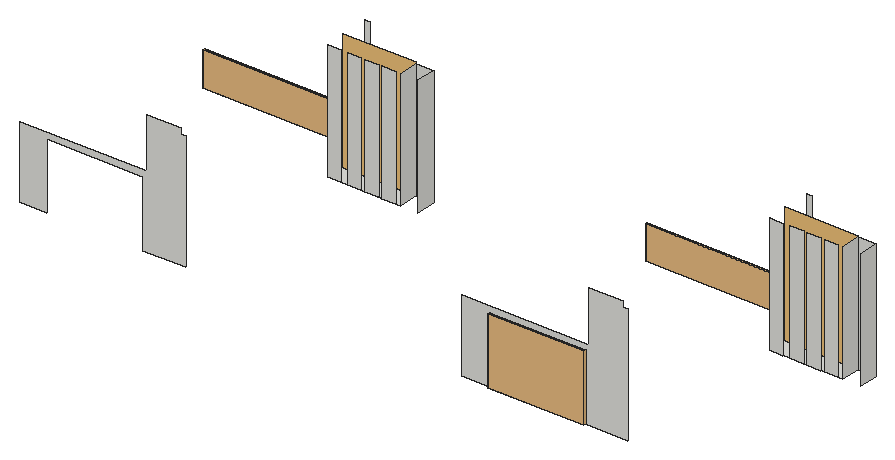
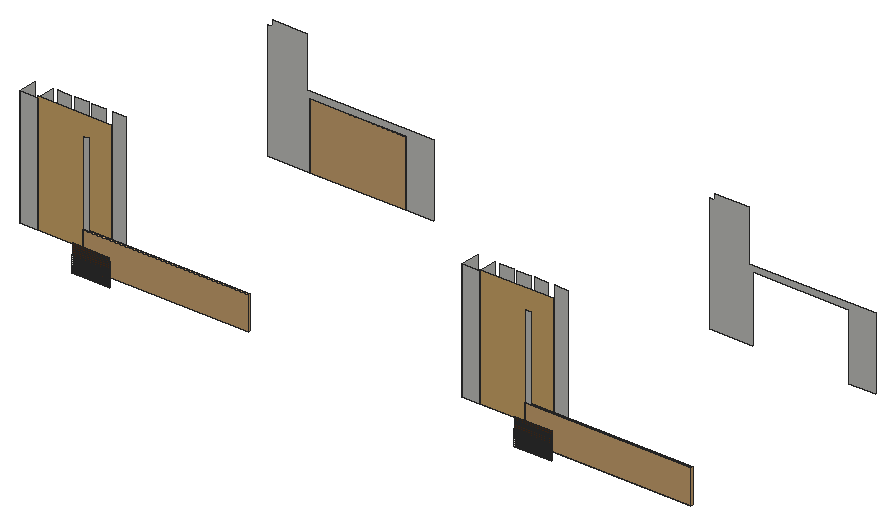
# SketchUp Ruby script. Lengths in inches.
U = 1.inch
M = Sketchup.active_model
def pt(a) = Geom::Point3d.new(a.map { |v| v * U })
def face(e, loops, mat)
  f = e.add_face(loops[0].map { |a| pt(a) })
  loops[1..].each { |l| e.add_face(l.map { |a| pt(a) }).erase! }
  f.material = f.back_material = mat if mat
  f
end
# faces: each face lists its corners as indices into pts; further lists are holes
def faces(e, pts, list, mat = nil) = list.each { |f| face(e, (f[0].is_a?(Array) ? f : [f]).map { |l| l.map { |i| pts[i] } }, mat) }
# xy, xz, yz: faces in a plane at the given z, y or x. An outline is a flat list of corners, or four numbers for a rectangle; further outlines are holes
def ring(l) = l.size == 4 ? [[l[0], l[1]], [l[2], l[1]], [l[2], l[3]], [l[0], l[3]]] : l.each_slice(2).to_a
def flat(e, list, mat, &to3) = list.each { |f| face(e, (f[0].is_a?(Array) ? f : [f]).map { |l| ring(l).map { |u, v| to3.(u, v) } }, mat) }
def xy(e, z, list, mat = nil) = flat(e, list, mat) { |x, y| [x, y, z] }
def xz(e, y, list, mat = nil) = flat(e, list, mat) { |x, z| [x, y, z] }
def yz(e, x, list, mat = nil) = flat(e, list, mat) { |y, z| [x, y, z] }
def lines(e, pts, list) = list.each { |a, b| e.add_line(pt(pts[a]), pt(pts[b])) }
# prism: a flat outline (further loops are holes) pulled along v
def prism(e, loops, v, mat = nil)
  f = face(e, loops, mat); d = Geom::Vector3d.new(v.map { |x| x * U })
  f.pushpull(f.normal.samedirection?(d) ? d.length : -d.length)
end
def box(e, o, s, mat = nil) = prism(e, [[o, [o[0] + s[0], o[1], o[2]], [o[0] + s[0], o[1] + s[1], o[2]], [o[0], o[1] + s[1], o[2]]]], [0, 0, s[2]], mat)
def at(x, y, z, deg = 0) = Geom::Transformation.translation(pt([x, y, z])) * Geom::Transformation.rotation(ORIGIN, Z_AXIS, deg.degrees)
def axes(o, x, y, z) = Geom::Transformation.new([*x, 0, *y, 0, *z, 0, *pt(o).to_a, 1])
def part(name) = M.definitions.add(name)
# library, detail: a bought-in or finely detailed component or shape, given as its bounding box
def library(name, o, s) = part(name).tap { |d| box(d.entities, o, s) }
def detail(e, o, s) = box(e.add_group.entities, o, s)
def put(e, d, t, mat = nil) = e.add_instance(d, t).tap { |i| i.material = mat if mat }
def group(e, t, mat = nil) = e.add_group.tap { |g| g.transformation = t; g.material = mat if mat }.entities
root = M.entities
M.materials.add("[Wood OSB]1").color = [240, 195, 122]
M.materials.add("[Wood Veneer 01]").color = [96, 56, 29]
c1 = library("panneau+shadow+blanc+bourdon+naturel",[-47.99,-1.29,1.53],[97.82,5.86,114.18])
c2 = library("Glass Railing",[0,0,0],[139.5,4.76,42])
xy(root,195.63,[[609,982.06,782.4375,1027.68],[1657.31,982.06,1830.75,1027.68]])
xy(root,206.47,[[533.89,1125.04,620.51,1127.73],[1582.21,1125.04,1668.82,1127.73]])
xy(root,207.375,[[533.89,1125.04,620.51,1127.73],[1582.21,1125.04,1668.82,1127.73]])
xy(root,210.41,[[533.89,1125.04,620.51,1127.73],[1582.21,1125.04,1668.82,1127.73]])
xy(root,211.375,[[533.89,1125.04,620.51,1127.73],[1582.21,1125.04,1668.82,1127.73]])
xy(root,214.41,[[533.89,1125.04,620.51,1127.73],[1582.21,1125.04,1668.82,1127.73]])
xy(root,215.4375,[[533.89,1125.04,620.51,1127.73],[1582.21,1125.04,1668.82,1127.73]])
xy(root,218.47,[[533.89,1125.04,620.51,1127.73],[1582.21,1125.04,1668.82,1127.73]])
xy(root,219.5,[[533.89,1125.04,620.51,1127.73],[1582.21,1125.04,1668.82,1127.73]])
xy(root,222.53,[[533.89,1125.04,620.51,1127.73],[1582.21,1125.04,1668.82,1127.73]])
xy(root,223.5625,[[533.89,1125.04,620.51,1127.73],[1582.21,1125.04,1668.82,1127.73]])
xy(root,226.59,[[533.89,1125.04,620.51,1127.73],[1582.21,1125.04,1668.82,1127.73]])
xy(root,227.625,[[533.89,1125.04,620.51,1127.73],[1582.21,1125.04,1668.82,1127.73]])
xy(root,230.66,[[533.89,1125.04,620.51,1127.73],[1582.21,1125.04,1668.82,1127.73]])
xy(root,231.6875,[[533.89,1125.04,620.51,1127.73],[1582.21,1125.04,1668.82,1127.73]])
xy(root,234.72,[[533.89,1125.04,620.51,1127.73],[1582.21,1125.04,1668.82,1127.73]])
xy(root,235.75,[[533.89,1125.04,620.51,1127.73],[1582.21,1125.04,1668.82,1127.73]])
xy(root,238.78,[[533.89,1125.04,620.51,1127.73],[1582.21,1125.04,1668.82,1127.73]])
xy(root,239.8125,[[533.89,1125.04,620.51,1127.73],[1582.21,1125.04,1668.82,1127.73]])
xy(root,242.84,[[533.89,1125.04,620.51,1127.73],[1582.21,1125.04,1668.82,1127.73]])
xz(root,546.92,[[228.06,199,228.06,370.64,528.37,370.64,528.37,491.07,609.34,491.07,609.34,478.09,620.86,478.09,620.86,199,520.24,199,520.24,355.625,292.8,355.625,292.8,199],[1276.37,199,1276.37,370.64,1576.68,370.64,1576.68,491.07,1657.65,491.07,1657.65,478.09,1669.17,478.09,1669.17,199,1568.55,199,1568.55,355.625,1341.11,355.625,1341.11,199]])
xz(root,982.06,[[609,195.63,641.2,476.38],[656.68,195.63,688.89,476.38],[698.31,195.63,730.52,476.38],[738.93,195.63,771.14,476.38],[1657.31,195.63,1689.52,476.38],
  [1705,195.63,1737.2,476.38],[1746.62,195.63,1778.83,476.38],[1787.25,195.63,1819.45,476.38]])
xz(root,1027.68,[[782.4375,195.63,824.1875,476.38],[1830.75,195.63,1872.5,476.38]])
xz(root,1027.68,[[609,195.63,782.4375,480],[1657.31,195.63,1830.75,480]],"[Wood OSB]1")
xz(root,1092.87,[[609,203.4375,620.51,480],[1657.31,203.4375,1668.82,480]])
xz(root,1125.04,[[533.89,203.4375,620.51,206.47],[1582.21,203.4375,1668.82,206.47],[533.89,207.375,620.51,210.41],[1582.21,207.375,1668.82,210.41],[533.89,211.375,620.51,214.41],
  [1582.21,211.375,1668.82,214.41],[533.89,215.4375,620.51,218.47],[1582.21,215.4375,1668.82,218.47],[533.89,219.5,620.51,222.53],[1582.21,219.5,1668.82,222.53],
  [533.89,223.5625,620.51,226.59],[1582.21,223.5625,1668.82,226.59],[533.89,227.625,620.51,230.66],[1582.21,227.625,1668.82,230.66],[533.89,231.6875,620.51,234.72],
  [1582.21,231.6875,1668.82,234.72],[533.89,235.75,620.51,238.78],[1582.21,235.75,1668.82,238.78],[533.89,239.8125,620.51,242.84],[1582.21,239.8125,1668.82,242.84],
  [533.89,243.875,620.51,246.91],[1582.21,243.875,1668.82,246.91],[533.89,247.9375,620.51,250.97],[1582.21,247.9375,1668.82,250.97],[533.89,252,620.51,255.03],
  [1582.21,252,1668.82,255.03],[533.89,256.0625,620.51,259.09],[1582.21,256.0625,1668.82,259.09]],"[Wood Veneer 01]")
xz(root,1125.42,[[533.89,260.125,620.51,263.16],[1582.21,260.125,1668.82,263.16],[533.89,264.1875,620.51,267.22],[1582.21,264.1875,1668.82,267.22]],"[Wood Veneer 01]")
yz(root,782.4375,[[982.06,195.63,1027.68,476.38]])
yz(root,824.1875,[[982.06,195.63,1027.68,476.38]])
yz(root,1830.75,[[982.06,195.63,1027.68,476.38]])
yz(root,1872.5,[[982.06,195.63,1027.68,476.38]])
put(root,c1,axes([1452.7,543.34,196.89],[2.32508,0,0],[0,1,0],[0,0,1.37182]))
put(root,c2,axes([227.71,1090.45,203.38],[2.81576,0,0],[0,1,0],[0,0,1.9]))
put(root,c2,axes([1276.02,1090.45,203.38],[2.81576,0,0],[0,1,0],[0,0,1.9]))
